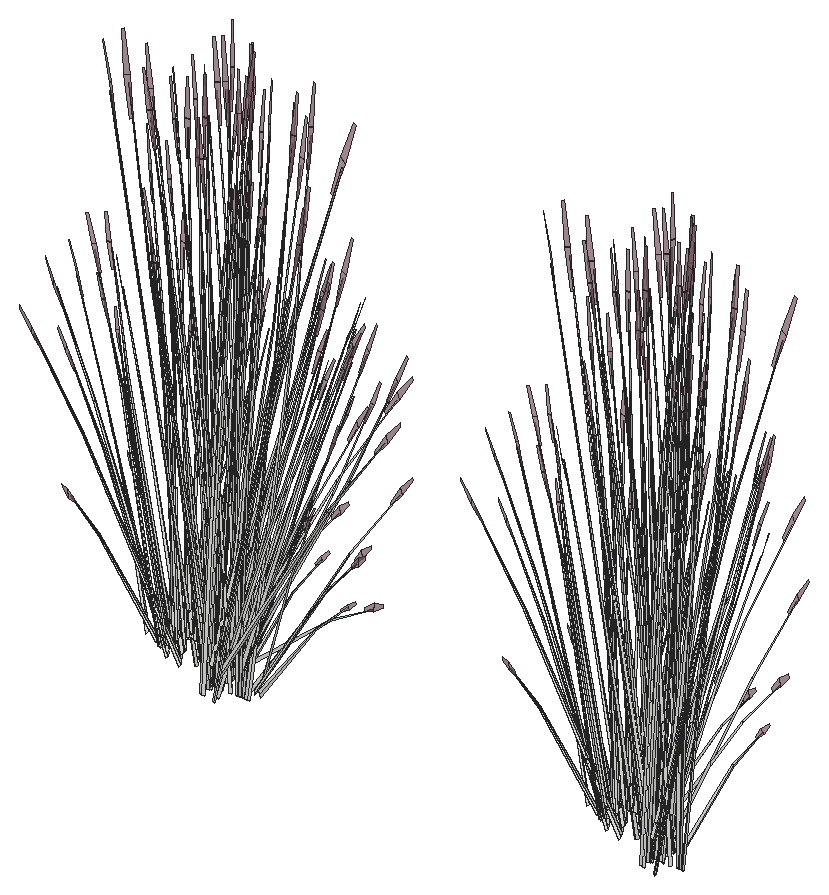
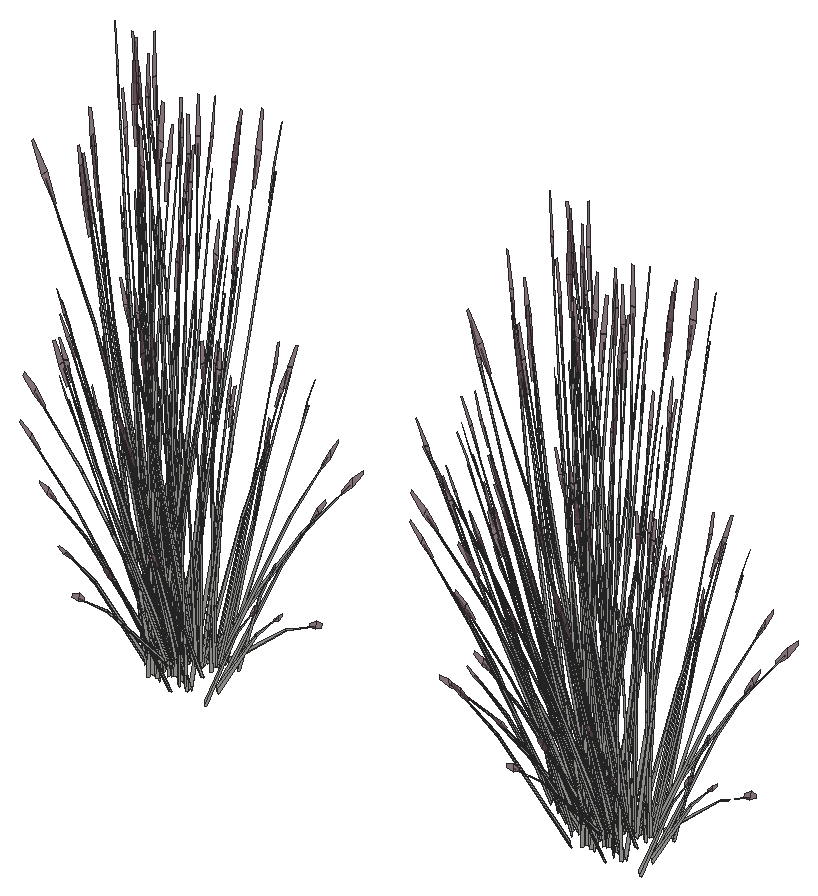
# SketchUp Ruby script. Lengths in inches.
U = 1.inch
M = Sketchup.active_model
def pt(a) = Geom::Point3d.new(a.map { |v| v * U })
def face(e, loops, mat)
  f = e.add_face(loops[0].map { |a| pt(a) })
  loops[1..].each { |l| e.add_face(l.map { |a| pt(a) }).erase! }
  f.material = f.back_material = mat if mat
  f
end
# faces: each face lists its corners as indices into pts; further lists are holes
def faces(e, pts, list, mat = nil) = list.each { |f| face(e, (f[0].is_a?(Array) ? f : [f]).map { |l| l.map { |i| pts[i] } }, mat) }
# xy, xz, yz: faces in a plane at the given z, y or x. An outline is a flat list of corners, or four numbers for a rectangle; further outlines are holes
def ring(l) = l.size == 4 ? [[l[0], l[1]], [l[2], l[1]], [l[2], l[3]], [l[0], l[3]]] : l.each_slice(2).to_a
def flat(e, list, mat, &to3) = list.each { |f| face(e, (f[0].is_a?(Array) ? f : [f]).map { |l| ring(l).map { |u, v| to3.(u, v) } }, mat) }
def xy(e, z, list, mat = nil) = flat(e, list, mat) { |x, y| [x, y, z] }
def xz(e, y, list, mat = nil) = flat(e, list, mat) { |x, z| [x, y, z] }
def yz(e, x, list, mat = nil) = flat(e, list, mat) { |y, z| [x, y, z] }
def lines(e, pts, list) = list.each { |a, b| e.add_line(pt(pts[a]), pt(pts[b])) }
# prism: a flat outline (further loops are holes) pulled along v
def prism(e, loops, v, mat = nil)
  f = face(e, loops, mat); d = Geom::Vector3d.new(v.map { |x| x * U })
  f.pushpull(f.normal.samedirection?(d) ? d.length : -d.length)
end
def box(e, o, s, mat = nil) = prism(e, [[o, [o[0] + s[0], o[1], o[2]], [o[0] + s[0], o[1] + s[1], o[2]], [o[0], o[1] + s[1], o[2]]]], [0, 0, s[2]], mat)
def at(x, y, z, deg = 0) = Geom::Transformation.translation(pt([x, y, z])) * Geom::Transformation.rotation(ORIGIN, Z_AXIS, deg.degrees)
def axes(o, x, y, z) = Geom::Transformation.new([*x, 0, *y, 0, *z, 0, *pt(o).to_a, 1])
def part(name) = M.definitions.add(name)
# library, detail: a bought-in or finely detailed component or shape, given as its bounding box
def library(name, o, s) = part(name).tap { |d| box(d.entities, o, s) }
def detail(e, o, s) = box(e.add_group.entities, o, s)
def put(e, d, t, mat = nil) = e.add_instance(d, t).tap { |i| i.material = mat if mat }
def group(e, t, mat = nil) = e.add_group.tap { |g| g.transformation = t; g.material = mat if mat }.entities
root = M.entities
M.materials.add("LightPink_Translucent").color = [144, 107, 117]
M.materials["LightPink_Translucent"].alpha = 0.75
c1 = part("blade")
p = [[2.15,0.21,22],[0,0.17,0],[0.09,0.45,0],[2.18,0.31,22],[2.29,0.31,22],[0.38,0.45,0],
  [2.48,0.24,33],[2.49,0.24,33],[2.48,0.22,33]]
faces(c1.entities,p,[[0,1,2,3],[4,5,2,3],[6,3,4,7],[8,0,3,6]])
c2 = part("seeds")
p = [[0.3,-0.1,1.38],[-0.01,-0.03,1.59],[-0.01,-0.03,0.03],[0.14,-0.07,-0.07],[0.29,-0.03,3],[0.15,0.01,3.11]]
faces(c2.entities,p,[[0,1,2,3],[1,0,4,5]],"LightPink_Translucent")
c3 = part("blade with seeds")
put(c3.entities,c1,at(0,0,0))
put(c3.entities,c2,axes([2.4,0.25,30.99],[1.5799,-0.05474,1.17369],[-0.12525,1.92788,0.29478],[-0.07173,-0.02425,1.56792]))
put(root,c3,axes([737.56,480.5,3.24],[-0.49383,0.08678,0.08821],[-0.12194,-0.32295,0.17543],[0.04404,0.04705,0.80203]))
put(root,c3,axes([761.76,480.5,3.24],[-0.49383,0.08678,0.08821],[-0.12194,-0.32295,0.17543],[0.04404,0.04705,0.80203]))
put(root,c3,axes([737.86,481.18,3.9375],[-0.19062,0.00741,0.85688],[0.12645,-0.32094,0.06928],[0.27165,0.01985,0.36631]))
put(root,c3,axes([738.11,480.49,3.01],[0.10795,0.28489,-0.15489],[-0.42874,0.0809,0.15489],[0.08643,0.03285,0.69487]))
put(root,c3,axes([762.31,480.49,3.01],[0.10795,0.28489,-0.15489],[-0.42874,0.0809,0.15489],[0.08643,0.03285,0.69487]))
put(root,c3,axes([738.85,481.625,4.37],[0.16879,0.22293,0.03215],[-0.30779,0.10912,0.2531],[0.13568,-0.02153,0.38595]))
put(root,c3,axes([737.24,481.125,3.19],[-0.58084,-0.06889,0.24599],[0.11821,-0.38906,0.09653],[0.08488,0.03757,0.85407]))
put(root,c3,axes([761.45,481.125,3.19],[-0.58084,-0.06889,0.24599],[0.11821,-0.38906,0.09653],[0.08488,0.03757,0.85407]))
put(root,c3,axes([738.8125,481.55,4.37],[-0.12984,0.29812,0.24001],[-0.42685,-0.10194,0.1979],[0.16786,-0.01792,0.49665]))
put(root,c3,axes([736.78,482.09,3.1],[-0.14994,-0.28188,0],[0.42817,-0.09871,0],[0,0,0.77185]))
put(root,c3,axes([760.98,482.09,3.1],[-0.14994,-0.28188,0],[0.42817,-0.09871,0],[0,0,0.77185]))
put(root,c3,axes([736.5,481.82,3.31],[-0.08866,0.29179,0.0724],[-0.43315,-0.05065,-0.20674],[-0.07883,-0.02996,0.63372]))
put(root,c3,axes([760.7,481.82,3.31],[-0.08866,0.29179,0.0724],[-0.43315,-0.05065,-0.20674],[-0.07883,-0.02996,0.63372]))
put(root,c3,axes([734.82,481.06,4.53],[0.38192,0.09121,0.17707],[-0.11139,0.2661,-0.2286],[-0.15377,0.0244,0.4374]))
put(root,c3,axes([759.02,481.06,4.53],[0.38192,0.09121,0.17707],[-0.11139,0.2661,-0.2286],[-0.15377,0.0244,0.4374]))
put(root,c3,axes([737.34,482.05,3.09],[0.48247,-0.11094,-0.09599],[0.16954,0.31956,0.00004],[0.05326,-0.01226,0.86949]))
put(root,c3,axes([761.54,482.05,3.09],[0.48247,-0.11094,-0.09599],[0.16954,0.31956,0.00004],[0.05326,-0.01226,0.86949]))
put(root,c3,axes([737.51,482.18,3.24],[0.13276,-0.32494,0.08821],[0.4858,0.09195,0.17543],[-0.08392,0.00158,0.80203]))
put(root,c3,axes([761.71,482.18,3.24],[0.13276,-0.32494,0.08821],[0.4858,0.09195,0.17543],[-0.08392,0.00158,0.80203]))
put(root,c3,axes([737.4,481.44,3.11],[0.32079,0.21119,0],[-0.32079,0.21119,0],[0,0,0.84633]))
put(root,c3,axes([761.6,481.44,3.11],[0.32079,0.21119,0],[-0.32079,0.21119,0],[0,0,0.84633]))
put(root,c3,axes([735.58,481.05,3.67],[0.13063,-0.0473,0.88532],[0.04505,0.33024,0.06928],[-0.28294,0.04382,0.31642]))
put(root,c3,axes([759.78,481.05,3.67],[0.13063,-0.0473,0.88532],[0.04505,0.33024,0.06928],[-0.28294,0.04382,0.31642]))
put(root,c3,axes([738.27,481.35,3.24],[-0.36107,-0.23816,0.08821],[0.36387,-0.231,0.17543],[-0.03988,0.04864,0.80203]))
put(root,c3,axes([762.47,481.35,3.24],[-0.36107,-0.23816,0.08821],[0.36387,-0.231,0.17543],[-0.03988,0.04864,0.80203]))
put(root,c3,axes([737.6,480.99,3.03],[0.47805,0.0536,-0.31177],[-0.10088,0.33065,-0.08182],[0.14266,0.04007,0.68817]))
put(root,c3,axes([739.71,481.57,3.38],[-0.28394,0.05398,0.5743],[0.13365,-0.22308,0.42196],[0.15063,0.01526,0.12649]))
put(root,c3,axes([736.68,482.21,3.1],[-0.4633,-0.14679,0],[0.22297,-0.30501,0],[0,0,0.81353]))
put(root,c3,axes([760.88,482.21,3.1],[-0.4633,-0.14679,0],[0.22297,-0.30501,0],[0,0,0.81353]))
put(root,c3,axes([737.06,481.82,3.23],[-0.44875,-0.26316,-0.12596],[0.3776,-0.2955,0.27565],[-0.12084,0.03078,0.84108]))
put(root,c3,axes([761.26,481.82,3.23],[-0.44875,-0.26316,-0.12596],[0.3776,-0.2955,0.27565],[-0.12084,0.03078,0.84108]))
put(root,c3,axes([735.88,482.33,3.24],[0.4301,0.16348,0.24825],[-0.25708,0.29314,0],[-0.09796,-0.03723,0.78752]))
put(root,c3,axes([760.08,482.33,3.24],[0.4301,0.16348,0.24825],[-0.25708,0.29314,0],[-0.09796,-0.03723,0.78752]))
put(root,c3,axes([737.39,481.19,3.36],[0.22297,-0.29461,0.2237],[0.4633,0.14179,-0.10766],[0,0.06791,0.71822]))
put(root,c3,axes([761.6,481.19,3.36],[0.22297,-0.29461,0.2237],[0.4633,0.14179,-0.10766],[0,0.06791,0.71822]))
put(root,c3,axes([739.58,482.51,4.35],[-0.04155,-0.02862,0.88692],[0.0909,-0.30682,-0.08381],[0.16368,-0.0196,0.15695]))
put(root,c3,axes([734.17,481.27,4.36],[-0.07505,0.04245,0.87472],[0.00638,0.31015,-0.13834],[-0.17202,0.04033,0.07015]))
put(root,c3,axes([758.375,481.27,4.36],[-0.07505,0.04245,0.87472],[0.00638,0.31015,-0.13834],[-0.17202,0.04033,0.07015]))
put(root,c3,axes([737.31,481.36,3.15],[0,0.37813,-0.02818],[-0.57465,0,0],[0,0.01188,0.89684]))
put(root,c3,axes([761.51,481.36,3.15],[0,0.37813,-0.02818],[-0.57465,0,0],[0,0.01188,0.89684]))
put(root,c3,axes([734.67,481.23,4.34],[-0.1245,0.29741,-0.25549],[-0.42685,-0.10194,-0.1979],[-0.17186,0.02727,0.48886]))
put(root,c3,axes([758.875,481.23,4.34],[-0.1245,0.29741,-0.25549],[-0.42685,-0.10194,-0.1979],[-0.17186,0.02727,0.48886]))
put(root,c3,axes([734.65,480.97,4.52],[0.23123,0.29606,-0.0608],[-0.41039,0.14549,-0.33747],[-0.17294,0.03906,0.51278]))
put(root,c3,axes([758.86,480.97,4.52],[0.23123,0.29606,-0.0608],[-0.41039,0.14549,-0.33747],[-0.17294,0.03906,0.51278]))
put(root,c3,axes([737.35,481.1,3.11],[0.27607,0.27443,-0.2237],[-0.41817,0.19325,0.10766],[0.08934,0.03396,0.71822]))
put(root,c3,axes([761.55,481.1,3.11],[0.27607,0.27443,-0.2237],[-0.41817,0.19325,0.10766],[0.08934,0.03396,0.71822]))
put(root,c3,axes([739.22,482.26,3.96],[-0.08796,-0.27485,-0.01746],[0.41573,-0.06319,-0.07916],[0.08682,0.01742,0.26109]))
put(root,c3,axes([735.63,482.5,3.1875],[-0.28732,0.32763,0],[-0.4807,-0.18271,-0.25804],[-0.10948,-0.04161,0.81856]))
put(root,c3,axes([759.83,482.5,3.1875],[-0.28732,0.32763,0],[-0.4807,-0.18271,-0.25804],[-0.10948,-0.04161,0.81856]))
put(root,c3,axes([738.14,482.25,4.52],[0.02461,-0.33251,-0.0608],[0.4659,0.00909,-0.33747],[0.17944,0.0231,0.51278]))
put(root,c3,axes([738.57,481.36,3.24],[0,-0.32696,0.24825],[0.51416,0,0],[0,0.07447,0.78752]))
put(root,c3,axes([762.77,481.36,3.24],[0,-0.32696,0.24825],[0.51416,0,0],[0,0.07447,0.78752]))
put(root,c3,axes([737.28,481.6,3.36],[0.49904,-0.02018,0.2237],[0.04513,0.33504,-0.10766],[-0.08934,0.03396,0.71822]))
put(root,c3,axes([761.48,481.6,3.36],[0.49904,-0.02018,0.2237],[0.04513,0.33504,-0.10766],[-0.08934,0.03396,0.71822]))
put(root,c3,axes([737.59,481.26,3.31],[0.42817,-0.09535,0.0724],[0.14994,0.27228,-0.20674],[0,0.05992,0.63372]))
put(root,c3,axes([761.79,481.26,3.31],[0.42817,-0.09535,0.0724],[0.14994,0.27228,-0.20674],[0,0.05992,0.63372]))
put(root,c3,axes([738.07,482.12,4.53],[-0.26148,-0.20471,0.17707],[0.29857,-0.19378,-0.2286],[0.1517,0.02948,0.4374]))
put(root,c3,axes([736.83,481.77,3.11],[-0.49904,0.02018,-0.2237],[-0.04513,-0.33504,0.10766],[-0.08934,0.03396,0.71822]))
put(root,c3,axes([761.03,481.77,3.11],[-0.49904,0.02018,-0.2237],[-0.04513,-0.33504,0.10766],[-0.08934,0.03396,0.71822]))
put(root,c3,axes([739.18,481.93,3.3],[-0.11068,-0.08041,0.71501],[0.144,-0.26601,-0.15377],[0.22393,0.03604,0.3057]))
put(root,c3,axes([737.2,482.22,3.1],[0.4633,0.14679,0],[-0.22297,0.30501,0],[0,0,0.87477]))
put(root,c3,axes([761.4,482.22,3.1],[0.4633,0.14679,0],[-0.22297,0.30501,0],[0,0,0.87477]))
put(root,c3,axes([738.55,482.05,4.36],[0.09858,-0.00553,0.87472],[0.2704,-0.25401,-0.13834],[0.17535,0.03353,0.07015]))
put(root,c3,axes([737.39,482.54,3.1],[-0.28374,-0.32877,-0.02571],[0.4807,-0.18271,0.25804],[-0.11845,0.0313,0.81815]))
put(root,c3,axes([761.59,482.54,3.1],[-0.28374,-0.32877,-0.02571],[0.4807,-0.18271,0.25804],[-0.11845,0.0313,0.81815]))
put(root,c3,axes([737.29,481.75,3.31],[0.33952,0.19644,0.0724],[-0.2832,0.22163,-0.20674],[-0.07883,0.02996,0.63372]))
put(root,c3,axes([761.49,481.75,3.31],[0.33952,0.19644,0.0724],[-0.2832,0.22163,-0.20674],[-0.07883,0.02996,0.63372]))
put(root,c3,axes([734.6,481.8,4.37],[-0.11397,-0.30091,0.24001],[0.44709,-0.05222,0.1979],[-0.13177,0.07077,0.49665]))
put(root,c3,axes([758.81,481.8,4.37],[-0.11397,-0.30091,0.24001],[0.44709,-0.05222,0.1979],[-0.13177,0.07077,0.49665]))
put(root,c3,axes([734.52,481.74,4.37],[-0.31549,-0.13751,0.03215],[0.18368,-0.19581,0.2531],[-0.10115,0.06331,0.38595]))
put(root,c3,axes([758.72,481.74,4.37],[-0.31549,-0.13751,0.03215],[0.18368,-0.19581,0.2531],[-0.10115,0.06331,0.38595]))
put(root,c3,axes([734.66,481.38,3.9375],[0.15946,-0.06916,0.85688],[0.13424,0.31957,0.06928],[-0.25033,0.07223,0.36631]))
put(root,c3,axes([758.86,481.38,3.9375],[0.15946,-0.06916,0.85688],[0.13424,0.31957,0.06928],[-0.25033,0.07223,0.36631]))
put(root,c3,axes([738.16,482.09,4.49],[0.45939,0.00787,-0.35523],[-0.03085,0.3315,0.04287],[0.19462,0.03498,0.5025]))
put(root,c3,axes([737.65,482.35,3.24],[0.4301,-0.16348,0.24825],[0.25708,0.29314,0],[-0.09796,0.03723,0.78752]))
put(root,c3,axes([761.85,482.35,3.24],[0.4301,-0.16348,0.24825],[0.25708,0.29314,0],[-0.09796,0.03723,0.78752]))
put(root,c3,axes([737.03,482.1,3.15],[0.1998,0.37562,-0.03006],[-0.5709,0.13162,0],[0.00698,0.01312,0.86086]))
put(root,c3,axes([761.24,482.1,3.15],[0.1998,0.37562,-0.03006],[-0.5709,0.13162,0],[0.00698,0.01312,0.86086]))
put(root,c3,axes([737.26,482.5,3.01],[-0.42874,-0.0809,-0.15489],[0.10795,-0.28489,0.15489],[-0.08643,0.03285,0.69487]))
put(root,c3,axes([761.46,482.5,3.01],[-0.42874,-0.0809,-0.15489],[0.10795,-0.28489,0.15489],[-0.08643,0.03285,0.69487]))
put(root,c3,axes([734.16,481.92,3.3],[0.15971,0.02684,0.71501],[0.10294,0.27415,-0.15377],[-0.21694,0.05132,0.3057]))
put(root,c3,axes([758.36,481.92,3.3],[0.15971,0.02684,0.71501],[0.10294,0.27415,-0.15377],[-0.21694,0.05132,0.3057]))
put(root,c3,axes([734.88,481.7,4.53],[0.40003,-0.04673,0.17707],[0.10563,0.26712,-0.2286],[-0.11464,0.07175,0.4374]))
put(root,c3,axes([759.08,481.7,4.53],[0.40003,-0.04673,0.17707],[0.10563,0.26712,-0.2286],[-0.11464,0.07175,0.4374]))
put(root,c3,axes([738.91,481.41,3.1875],[0.57465,0,0],[0,0.36542,-0.25804],[0,0.08323,0.81856]))
put(root,c3,axes([733.34,481.58,4.35],[0.05865,0.00877,0.88692],[0.18143,0.28888,-0.08381],[-0.12006,0.07582,0.15695]))
put(root,c3,axes([757.54,481.58,4.35],[0.05865,0.00877,0.88692],[0.18143,0.28888,-0.08381],[-0.12006,0.07582,0.15695]))
put(root,c3,axes([738.68,481.6,3.1],[-0.57436,-0.00261,-0.02488],[0,-0.36542,0.24971],[-0.01805,0.08319,0.79176]))
put(root,c3,axes([762.89,481.6,3.1],[-0.57436,-0.00261,-0.02488],[0,-0.36542,0.24971],[-0.01805,0.08319,0.79176]))
put(root,c3,axes([737.44,481.28,3.33],[0.51755,0.15601,-0.14548],[-0.2492,0.32927,-0.25001],[0.01626,0.08084,0.79854]))
put(root,c3,axes([761.64,481.28,3.33],[0.51755,0.15601,-0.14548],[-0.2492,0.32927,-0.25001],[0.01626,0.08084,0.79854]))
put(root,c3,axes([733.83,482.5,3.38],[0.19152,-0.14818,0.5743],[0.07557,0.23459,0.42196],[-0.13841,0.042,0.12649]))
put(root,c3,axes([758.03,482.5,3.38],[0.19152,-0.14818,0.5743],[0.07557,0.23459,0.42196],[-0.13841,0.042,0.12649]))
put(root,c3,axes([738.44,482.22,4.26],[0.26148,0.20471,-0.17707],[-0.29857,0.19378,0.2286],[0.1517,0.02948,0.4374]))
put(root,c3,axes([738.57,481.66,3.01],[-0.32079,0.20399,-0.15489],[-0.32079,-0.20399,0.15489],[0,0.06571,0.69487]))
put(root,c3,axes([762.77,481.66,3.01],[-0.32079,0.20399,-0.15489],[-0.32079,-0.20399,0.15489],[0,0.06571,0.69487]))
put(root,c3,axes([737.18,481.68,3.33],[0.05355,0.37308,-0.14548],[-0.55775,0.02256,-0.25001],[-0.09822,0.04969,0.79854]))
put(root,c3,axes([761.38,481.68,3.33],[0.05355,0.37308,-0.14548],[-0.55775,0.02256,-0.25001],[-0.09822,0.04969,0.79854]))
put(root,c3,axes([738.31,482.3,4.37],[-0.02314,0.24862,0.03215],[-0.34943,-0.00682,0.2531],[0.13385,0.02602,0.38595]))
put(root,c3,axes([737.39,481.53,3.11],[-0.22297,0.29461,-0.2237],[-0.4633,-0.14179,0.10766],[0,0.06791,0.71822]))
put(root,c3,axes([761.59,481.53,3.11],[-0.22297,0.29461,-0.2237],[-0.4633,-0.14179,0.10766],[0,0.06791,0.71822]))
put(root,c3,axes([734.55,481.86,4.26],[-0.40003,0.04673,-0.17707],[-0.10563,-0.26712,0.2286],[-0.11464,0.07175,0.4374]))
put(root,c3,axes([758.75,481.86,4.26],[-0.40003,0.04673,-0.17707],[-0.10563,-0.26712,0.2286],[-0.11464,0.07175,0.4374]))
put(root,c3,axes([738.34,482.22,4.37],[-0.33886,0.21544,0.24001],[-0.29224,-0.22879,0.1979],[0.15898,0.03974,0.49665]))
put(root,c3,axes([733.97,482.46,4.82],[0.40553,0.08728,-0.03244],[-0.12475,0.26862,-0.14708],[-0.06633,0.04078,0.48512]))
put(root,c3,axes([758.17,482.46,4.82],[0.40553,0.08728,-0.03244],[-0.12475,0.26862,-0.14708],[-0.06633,0.04078,0.48512]))
put(root,c3,axes([736.85,481.96,3.03],[-0.30954,0.24575,-0.31177],[-0.38452,-0.22284,-0.08182],[-0.12404,0.0613,0.68817]))
put(root,c3,axes([761.05,481.96,3.03],[-0.30954,0.24575,-0.31177],[-0.38452,-0.22284,-0.08182],[-0.12404,0.0613,0.68817]))
put(root,c3,axes([737.26,482.47,4.53],[-0.07098,-0.26335,0.17707],[0.40574,-0.06954,-0.2286],[0.10898,0.07547,0.4374]))
put(root,c3,axes([761.46,482.47,4.53],[-0.07098,-0.26335,0.17707],[0.40574,-0.06954,-0.2286],[0.10898,0.07547,0.4374]))
put(root,c3,axes([737.4,482.375,3.17],[0.57533,0.10627,0.15378],[-0.14394,0.37986,-0.18246],[-0.09522,0.04754,0.82443]))
put(root,c3,axes([761.6,482.375,3.17],[0.57533,0.10627,0.15378],[-0.14394,0.37986,-0.18246],[-0.09522,0.04754,0.82443]))
put(root,c3,axes([737.36,482.63,3.01],[-0.4301,0.16348,-0.24825],[-0.25708,-0.29314,0],[-0.09796,0.03723,0.78752]))
put(root,c3,axes([761.56,482.63,3.01],[-0.4301,0.16348,-0.24825],[-0.25708,-0.29314,0],[-0.09796,0.03723,0.78752]))
put(root,c3,axes([738.79,481.66,3.01],[0,0.32696,-0.24825],[-0.51416,0,0],[0,0.07447,0.78752]))
put(root,c3,axes([762.99,481.66,3.01],[0,0.32696,-0.24825],[-0.51416,0,0],[0,0.07447,0.78752]))
put(root,c3,axes([737.5,481.7,3.9375],[-0.1707,-0.05633,0.85688],[0.35326,-0.23632,0.06928],[0.22018,0.10661,0.36631]))
put(root,c3,axes([737.53,480.96,4.24],[-0.39711,-0.16988,0.69141],[0.41931,-0.2645,0.29833],[0.12812,0.1594,0.66832]))
put(root,c3,axes([761.74,480.96,4.24],[-0.39711,-0.16988,0.69141],[0.41931,-0.2645,0.29833],[0.12812,0.1594,0.66832]))
put(root,c3,axes([734.67,481.67,4.52],[0.4251,0.18028,-0.0608],[-0.24491,0.26108,-0.33747],[-0.1201,0.09075,0.51278]))
put(root,c3,axes([758.875,481.67,4.52],[0.4251,0.18028,-0.0608],[-0.24491,0.26108,-0.33747],[-0.1201,0.09075,0.51278]))
put(root,c3,axes([738.13,482.34,3.38],[-0.25875,-0.09401,0.5743],[0.33411,-0.09552,0.42196],[0.09012,0.08091,0.12649]))
put(root,c3,axes([762.33,482.34,3.38],[-0.25875,-0.09401,0.5743],[0.33411,-0.09552,0.42196],[0.09012,0.08091,0.12649]))
put(root,c3,axes([737.22,482.61,4.52],[0.27385,-0.27986,-0.0608],[0.39658,0.16123,-0.33747],[0.13785,0.07907,0.51278]))
put(root,c3,axes([735.24,481.59,3.9375],[0.11478,-0.10046,0.85688],[0.28982,0.27117,0.06928],[-0.19878,0.12349,0.36631]))
put(root,c3,axes([759.45,481.59,3.9375],[0.11478,-0.10046,0.85688],[0.28982,0.27117,0.06928],[-0.19878,0.12349,0.36631]))
put(root,c3,axes([734.88,481.89,4.34],[0.11806,0.29854,-0.25549],[-0.44709,0.05222,-0.1979],[-0.12812,0.08019,0.48886]))
put(root,c3,axes([759.08,481.89,4.34],[0.11806,0.29854,-0.25549],[-0.44709,0.05222,-0.1979],[-0.12812,0.08019,0.48886]))
put(root,c3,axes([735.42,482.23,4.53],[0.31095,-0.17214,0.17707],[0.29435,0.19656,-0.2286],[-0.04479,0.09987,0.4374]))
put(root,c3,axes([759.62,482.23,4.53],[0.31095,-0.17214,0.17707],[0.29435,0.19656,-0.2286],[-0.04479,0.09987,0.4374]))
put(root,c3,axes([737.75,482.58,3.1875],[0.28732,0.32763,0],[-0.4807,0.18271,-0.25804],[-0.10948,0.04161,0.81856]))
put(root,c3,axes([761.95,482.58,3.1875],[0.28732,0.32763,0],[-0.4807,0.18271,-0.25804],[-0.10948,0.04161,0.81856]))
put(root,c3,axes([736.87,482.84,4.35],[0.00136,-0.03958,0.88692],[0.39383,-0.17464,-0.08381],[0.1368,0.06234,0.15695]))
put(root,c3,axes([761.07,482.84,4.35],[0.00136,-0.03958,0.88692],[0.39383,-0.17464,-0.08381],[0.1368,0.06234,0.15695]))
put(root,c3,axes([738.21,482.69,2.75],[0.03348,-0.0472,0.88171],[0.42153,-0.13902,-0.1347],[0.12779,0.07195,0.15018]))
put(root,c3,axes([737.5,481.28,3.42],[-0.01255,-0.30784,0.70636],[0.56816,0.0798,0.29908],[-0.13438,0.16845,0.66675]))
put(root,c3,axes([761.7,481.28,3.42],[-0.01255,-0.30784,0.70636],[0.56816,0.0798,0.29908],[-0.13438,0.16845,0.66675]))
put(root,c3,axes([737.65,481.62,3.05],[0.16851,0.29936,-0.34606],[-0.4854,0.10781,-0.09083],[0.01863,0.10137,0.76386]))
put(root,c3,axes([761.85,481.62,3.05],[0.16851,0.29936,-0.34606],[-0.4854,0.10781,-0.09083],[0.01863,0.10137,0.76386]))
put(root,c3,axes([735.14,482.39,4.37],[-0.37765,-0.01523,0.03215],[0.01035,-0.23004,0.2531],[-0.03952,0.08812,0.38595]))
put(root,c3,axes([759.34,482.39,4.37],[-0.37765,-0.01523,0.03215],[0.01035,-0.23004,0.2531],[-0.03952,0.08812,0.38595]))
put(root,c3,axes([734.33,482.65,2.75],[0.06164,0.03267,0.88171],[0.10452,0.30266,-0.1347],[-0.13662,0.06454,0.15018]))
put(root,c3,axes([758.54,482.65,2.75],[0.06164,0.03267,0.88171],[0.10452,0.30266,-0.1347],[-0.13662,0.06454,0.15018]))
put(root,c3,axes([735.26,482.41,4.37],[-0.32725,-0.22308,0.24001],[0.34753,-0.1924,0.1979],[-0.06036,0.10466,0.49665]))
put(root,c3,axes([759.46,482.41,4.37],[-0.32725,-0.22308,0.24001],[0.34753,-0.1924,0.1979],[-0.06036,0.10466,0.49665]))
put(root,c3,axes([737.55,482.47,4.34],[0.45348,-0.07772,-0.25549],[0.07933,0.29434,-0.1979],[0.1218,0.08435,0.48886]))
put(root,c3,axes([736.29,482.51,4.53],[0.13855,-0.25143,0.17707],[0.4042,0.07334,-0.2286],[0.03706,0.10123,0.4374]))
put(root,c3,axes([760.49,482.51,4.53],[0.13855,-0.25143,0.17707],[0.4042,0.07334,-0.2286],[0.03706,0.10123,0.4374]))
put(root,c3,axes([738.17,482.77,3.33],[-0.2947,-0.01025,0.5253],[0.19462,-0.21779,0.29003],[0.11642,0.07737,0.41205]))
put(root,c3,axes([737.33,482.71,4.37],[-0.20887,0.2077,0.03215],[-0.29744,-0.12092,0.2531],[0.09616,0.06659,0.38595]))
put(root,c3,axes([761.53,482.71,4.37],[-0.20887,0.2077,0.03215],[-0.29744,-0.12092,0.2531],[0.09616,0.06659,0.38595]))
put(root,c3,axes([736.83,483.41,4.82],[0.31757,-0.18757,-0.03244],[0.29098,0.20543,-0.14708],[0.02049,0.05821,0.48512]))
put(root,c3,axes([761.04,483.41,4.82],[0.31757,-0.18757,-0.03244],[0.29098,0.20543,-0.14708],[0.02049,0.05821,0.48512]))
put(root,c3,axes([737.41,482.65,4.37],[-0.45708,0.07503,0.24001],[-0.07933,-0.29434,0.1979],[0.1075,0.08675,0.49665]))
put(root,c3,axes([761.61,482.65,4.37],[-0.45708,0.07503,0.24001],[-0.07933,-0.29434,0.1979],[0.1075,0.08675,0.49665]))
put(root,c3,axes([735.16,481.84,3.9375],[0.08557,-0.11238,0.85688],[0.35897,0.23257,0.06928],[-0.16194,0.14495,0.36631]))
put(root,c3,axes([759.36,481.84,3.9375],[0.08557,-0.11238,0.85688],[0.35897,0.23257,0.06928],[-0.16194,0.14495,0.36631]))
put(root,c3,axes([737.21,482.24,3.3],[0.00811,-0.10838,0.71501],[0.38755,-0.12106,-0.15377],[0.11964,0.12972,0.3057]))
put(root,c3,axes([761.41,482.24,3.3],[0.00811,-0.10838,0.71501],[0.38755,-0.12106,-0.15377],[0.11964,0.12972,0.3057]))
put(root,c3,axes([736.17,482.74,4.37],[-0.33863,0.11112,0.03215],[-0.16575,-0.20263,0.2531],[0.0327,0.08932,0.38595]))
put(root,c3,axes([760.37,482.74,4.37],[-0.33863,0.11112,0.03215],[-0.16575,-0.20263,0.2531],[0.0327,0.08932,0.38595]))
put(root,c3,axes([735.26,482.48,4.26],[-0.31095,0.17214,-0.17707],[-0.29435,-0.19656,0.2286],[-0.04479,0.09987,0.4374]))
put(root,c3,axes([759.46,482.48,4.26],[-0.31095,0.17214,-0.17707],[-0.29435,-0.19656,0.2286],[-0.04479,0.09987,0.4374]))
put(root,c3,axes([734.18,482.42,4.36],[-0.01142,0.0647,0.87472],[0.32418,0.22509,-0.13834],[-0.08487,0.10644,0.07015]))
put(root,c3,axes([758.39,482.42,4.36],[-0.01142,0.0647,0.87472],[0.32418,0.22509,-0.13834],[-0.08487,0.10644,0.07015]))
put(root,c3,axes([735.22,482.28,4.7],[0.50507,0.0162,-0.06749],[-0.01381,0.30672,-0.3746],[-0.03508,0.11813,0.56919]))
put(root,c3,axes([759.42,482.28,4.7],[0.50507,0.0162,-0.06749],[-0.01381,0.30672,-0.3746],[-0.03508,0.11813,0.56919]))
put(root,c3,axes([736.16,482.62,4.52],[0.44971,-0.15222,-0.0608],[0.221,0.27017,-0.33747],[0.05933,0.11385,0.51278]))
put(root,c3,axes([760.36,482.62,4.52],[0.44971,-0.15222,-0.0608],[0.221,0.27017,-0.33747],[0.05933,0.11385,0.51278]))
put(root,c3,axes([736.29,482.72,4.53],[-0.45283,-0.08548,0.26641],[0.15485,-0.28101,0.21967],[0.02721,0.11051,0.55128]))
put(root,c3,axes([760.49,482.72,4.53],[-0.45283,-0.08548,0.26641],[0.15485,-0.28101,0.21967],[0.02721,0.11051,0.55128]))
put(root,c3,axes([735.45,483.14,3.38],[-0.01189,-0.19441,0.5743],[0.29719,0.13866,0.42196],[-0.05845,0.09266,0.12649]))
put(root,c3,axes([759.66,483.14,3.38],[-0.01189,-0.19441,0.5743],[0.29719,0.13866,0.42196],[-0.05845,0.09266,0.12649]))
put(root,c3,axes([736.24,482.68,2.75],[0.07437,-0.01779,0.88171],[0.44738,0.09793,-0.1347],[0.01308,0.11037,0.15018]))
put(root,c3,axes([760.4375,482.68,2.75],[0.07437,-0.01779,0.88171],[0.44738,0.09793,-0.1347],[0.01308,0.11037,0.15018]))
put(root,c3,axes([735.57,482.39,4.5],[0.32898,0.21969,-0.2836],[-0.34753,0.1924,-0.21967],[-0.05006,0.11162,0.54264]))
put(root,c3,axes([759.77,482.39,4.5],[0.32898,0.21969,-0.2836],[-0.34753,0.1924,-0.21967],[-0.05006,0.11162,0.54264]))
put(root,c3,axes([735.21,482.72,3.41],[0.41748,-0.0579,0.03254],[0.09598,0.23326,-0.43152],[-0.02647,0.11808,0.3868]))
put(root,c3,axes([759.41,482.72,3.41],[0.41748,-0.0579,0.03254],[0.09598,0.23326,-0.43152],[-0.02647,0.11808,0.3868]))
put(root,c3,axes([736.54,482.61,4.34],[0.45175,0.08196,-0.25549],[-0.15485,0.28101,-0.1979],[0.04142,0.11314,0.48886]))
put(root,c3,axes([760.74,482.61,4.34],[0.45175,0.08196,-0.25549],[-0.15485,0.28101,-0.1979],[0.04142,0.11314,0.48886]))
put(root,c3,axes([736.8,482.03,3.9375],[-0.10505,-0.10498,0.85688],[0.48542,-0.08838,0.06928],[0.10971,0.1648,0.36631]))
put(root,c3,axes([761,482.03,3.9375],[-0.10505,-0.10498,0.85688],[0.48542,-0.08838,0.06928],[0.10971,0.1648,0.36631]))
put(root,c3,axes([736.34,482.78,4.26],[-0.13855,0.25143,-0.17707],[-0.4042,-0.07334,0.2286],[0.03706,0.10123,0.4374]))
put(root,c3,axes([760.54,482.78,4.26],[-0.13855,0.25143,-0.17707],[-0.4042,-0.07334,0.2286],[0.03706,0.10123,0.4374]))
put(root,c3,axes([735.46,482.29,4.67],[-0.01196,0.30243,-0.3943],[-0.50354,-0.02031,0.04758],[-0.05314,0.12813,0.55778]))
put(root,c3,axes([759.67,482.29,4.67],[-0.01196,0.30243,-0.3943],[-0.50354,-0.02031,0.04758],[-0.05314,0.12813,0.55778]))
put(root,c3,axes([734.15,483.09,4.35],[0.05214,-0.01974,0.88692],[0.43092,0.1313,-0.08381],[-0.01013,0.10932,0.15695]))
put(root,c3,axes([758.35,483.09,4.35],[0.05214,-0.01974,0.88692],[0.43092,0.1313,-0.08381],[-0.01013,0.10932,0.15695]))
put(root,c3,axes([735.94,482.08,3.9375],[-0.01125,-0.12549,0.85688],[0.48751,0.08325,0.06928],[-0.03015,0.17883,0.36631]))
put(root,c3,axes([760.14,482.08,3.9375],[-0.01125,-0.12549,0.85688],[0.48751,0.08325,0.06928],[-0.03015,0.17883,0.36631]))
put(root,c3,axes([736.375,482.55,4.49],[0.21934,0.26585,-0.35523],[-0.45151,0.14816,0.04287],[0.05129,0.12845,0.5025]))
put(root,c3,axes([760.58,482.55,4.49],[0.21934,0.26585,-0.35523],[-0.45151,0.14816,0.04287],[0.05129,0.12845,0.5025]))
put(root,c3,axes([735.11,482.97,3.3],[0.14502,-0.05158,0.71501],[0.35805,0.15552,-0.15377],[-0.10657,0.13457,0.3057]))
put(root,c3,axes([759.31,482.97,3.3],[0.14502,-0.05158,0.71501],[0.35805,0.15552,-0.15377],[-0.10657,0.13457,0.3057]))
put(root,c3,axes([736.05,483.23,4.36],[0.05825,0.05265,0.87472],[0.47011,0.02068,-0.13834],[0.04727,0.11612,0.07015]))
put(root,c3,axes([760.25,483.23,4.36],[0.05825,0.05265,0.87472],[0.47011,0.02068,-0.13834],[0.04727,0.11612,0.07015]))
put(root,c3,axes([735.29,482.72,3.68],[0.0101,-0.16879,0.77173],[0.45413,0.08915,0.10664],[-0.03935,0.17989,0.36441]))
put(root,c3,axes([759.5,482.72,3.68],[0.0101,-0.16879,0.77173],[0.45413,0.08915,0.10664],[-0.03935,0.17989,0.36441]))
